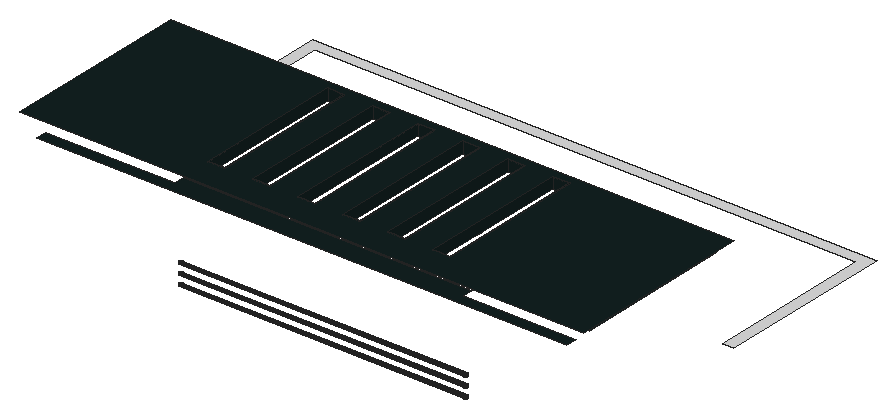
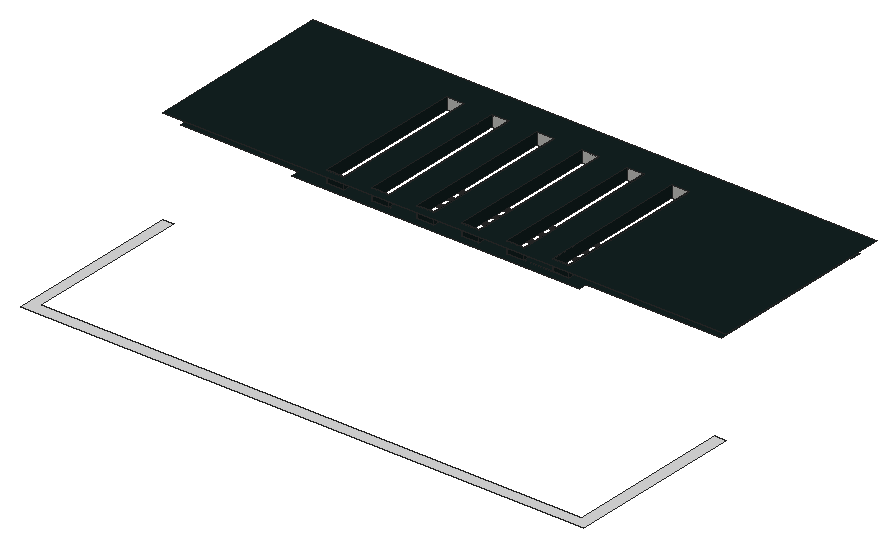
# SketchUp Ruby script. Lengths in millimetres.
U = 1.mm
M = Sketchup.active_model
def pt(a) = Geom::Point3d.new(a.map { |v| v * U })
def face(e, loops, mat)
  f = e.add_face(loops[0].map { |a| pt(a) })
  loops[1..].each { |l| e.add_face(l.map { |a| pt(a) }).erase! }
  f.material = f.back_material = mat if mat
  f
end
# faces: each face lists its corners as indices into pts; further lists are holes
def faces(e, pts, list, mat = nil) = list.each { |f| face(e, (f[0].is_a?(Array) ? f : [f]).map { |l| l.map { |i| pts[i] } }, mat) }
# xy, xz, yz: faces in a plane at the given z, y or x. An outline is a flat list of corners, or four numbers for a rectangle; further outlines are holes
def ring(l) = l.size == 4 ? [[l[0], l[1]], [l[2], l[1]], [l[2], l[3]], [l[0], l[3]]] : l.each_slice(2).to_a
def flat(e, list, mat, &to3) = list.each { |f| face(e, (f[0].is_a?(Array) ? f : [f]).map { |l| ring(l).map { |u, v| to3.(u, v) } }, mat) }
def xy(e, z, list, mat = nil) = flat(e, list, mat) { |x, y| [x, y, z] }
def xz(e, y, list, mat = nil) = flat(e, list, mat) { |x, z| [x, y, z] }
def yz(e, x, list, mat = nil) = flat(e, list, mat) { |y, z| [x, y, z] }
def lines(e, pts, list) = list.each { |a, b| e.add_line(pt(pts[a]), pt(pts[b])) }
# prism: a flat outline (further loops are holes) pulled along v
def prism(e, loops, v, mat = nil)
  f = face(e, loops, mat); d = Geom::Vector3d.new(v.map { |x| x * U })
  f.pushpull(f.normal.samedirection?(d) ? d.length : -d.length)
end
def box(e, o, s, mat = nil) = prism(e, [[o, [o[0] + s[0], o[1], o[2]], [o[0] + s[0], o[1] + s[1], o[2]], [o[0], o[1] + s[1], o[2]]]], [0, 0, s[2]], mat)
def at(x, y, z, deg = 0) = Geom::Transformation.translation(pt([x, y, z])) * Geom::Transformation.rotation(ORIGIN, Z_AXIS, deg.degrees)
def axes(o, x, y, z) = Geom::Transformation.new([*x, 0, *y, 0, *z, 0, *pt(o).to_a, 1])
def part(name) = M.definitions.add(name)
# library, detail: a bought-in or finely detailed component or shape, given as its bounding box
def library(name, o, s) = part(name).tap { |d| box(d.entities, o, s) }
def detail(e, o, s) = box(e.add_group.entities, o, s)
def put(e, d, t, mat = nil) = e.add_instance(d, t).tap { |i| i.material = mat if mat }
def group(e, t, mat = nil) = e.add_group.tap { |g| g.transformation = t; g.material = mat if mat }.entities
root = M.entities
M.materials.add("[0078_DarkSlateGray]").color = [19, 33, 33]
M.materials.add("[0128_White]").color = [252, 252, 252]
M.materials.add("[0130_Gainsboro]").color = [220, 220, 220]
xy(root,69967.5,[[7076.1,23710.9,7685.7,23710.9,7685.7,32702.5,36946.5,32702.5,36946.5,23710.9,37556.1,23710.9,37556.1,33312.1,7076.1,33312.1]],"[0130_Gainsboro]")
xy(root,74234.7,[[7990.5,13550.9,7990.5,14109.7,15000.9,14109.7,15000.9,14719.3,30545.7,14719.3,30545.7,14109.7,36641.7,14109.7,36641.7,13550.9]],"[0078_DarkSlateGray]")
xy(root,74539.5,[[[7685.7,14719.3,7685.7,23253.7,15915.3,23253.7,15915.3,15176.5,16829.7,15176.5,16829.7,23253.7,18353.7,23253.7,18353.7,15176.5,19268.1,15176.5,19268.1,23253.7,20792.1,23253.7,20792.1,15176.5,21706.5,15176.5,21706.5,23253.7,23230.5,23253.7,23230.5,15176.5,24144.9,15176.5,24144.9,23253.7,25668.9,23253.7,25668.9,15176.5,26583.3,15176.5,26583.3,23253.7,28107.3,23253.7,28107.3,15176.5,29021.7,15176.5,29021.7,23253.7,15000.9,23253.7,15000.9,23710.9,30545.7,23710.9,30545.7,23253.7,36946.5,23253.7,36946.5,14719.3],[17596.1,17794.4,17659.9,17796.3,17723.1,17804.9,17785.1,17820.1,17845.1,17841.6,17902.6,17869.3,17956.9,17902.9,18007.3,17942,18053.4,17986.1,18094.7,18034.8,18130.6,18087.5,18160.8,18143.7,18185,18202.8,18202.8,18264,18214.2,18326.8,18218.9,18390.5,18217,18454.2,18208.4,18517.5,18193.2,18579.4,18171.7,18639.5,18143.9,18697,18110.4,18751.2,18071.3,18801.7,18027.2,18847.8,17978.5,18889,17925.8,18924.9,17869.6,18955.1,17810.5,18979.3,17749.2,18997.2,17686.5,19008.5,17622.8,19013.3,17559,19011.3,17495.8,19002.7,17433.8,18987.6,17373.8,18966,17316.3,18938.3,17262,18904.7,17211.6,18865.7,17165.5,18821.6,17124.3,18772.9,17088.3,18720.1,17058.1,18663.9,17034,18604.9,17016.1,18543.6,17004.7,18480.8,17000,18417.2,17001.9,18353.4,17010.5,18290.2,17025.7,18228.2,17047.3,18168.1,17075,18110.7,17108.5,18056.4,17147.6,18006,17191.7,17959.9,17240.4,17918.6,17293.2,17882.7,17349.4,17852.5,17408.4,17828.3,17469.7,17810.5,17532.5,17799.1],[20031.3,17794.4,20095.1,17796.3,20158.3,17804.9,20220.3,17820.1,20280.4,17841.6,20337.8,17869.3,20392.1,17902.9,20442.6,17942,20488.6,17986.1,20529.9,18034.8,20565.8,18087.5,20596,18143.7,20620.2,18202.8,20638,18264,20649.4,18326.8,20654.1,18390.5,20652.2,18454.2,20643.6,18517.5,20628.4,18579.4,20606.9,18639.5,20579.2,18697,20545.6,18751.2,20506.5,18801.7,20462.4,18847.8,20413.7,18889,20361,18924.9,20304.8,18955.1,20245.7,18979.3,20184.5,18997.2,20121.7,19008.5,20058,19013.3,19994.3,19011.3,19931,19002.7,19869.1,18987.6,19809,18966,19751.5,18938.3,19697.3,18904.7,19646.8,18865.7,19600.7,18821.6,19559.5,18772.9,19523.6,18720.1,19493.4,18663.9,19469.2,18604.9,19451.3,18543.6,19440,18480.8,19435.2,18417.2,19437.2,18353.4,19445.8,18290.2,19460.9,18228.2,19482.5,18168.1,19510.2,18110.7,19543.8,18056.4,19582.8,18006,19626.9,17959.9,19675.6,17918.6,19728.4,17882.7,19784.6,17852.5,19843.6,17828.3,19904.9,17810.5,19967.7,17799.1],[24972.2,17794.4,25036,17796.3,25099.2,17804.9,25161.2,17820.1,25221.3,17841.6,25278.7,17869.3,25333,17902.9,25383.5,17942,25429.6,17986.1,25470.8,18034.8,25506.7,18087.5,25536.9,18143.7,25561.1,18202.8,25578.9,18264,25590.3,18326.8,25595,18390.5,25593.1,18454.2,25584.5,18517.5,25569.3,18579.4,25547.8,18639.5,25520.1,18697,25486.5,18751.2,25447.4,18801.7,25403.3,18847.8,25354.6,18889,25301.9,18924.9,25245.7,18955.1,25186.6,18979.3,25125.4,18997.2,25062.6,19008.5,24999,19013.3,24935.2,19011.3,24872,19002.7,24810,18987.6,24749.9,18966,24692.4,18938.3,24638.2,18904.7,24587.7,18865.7,24541.6,18821.6,24500.4,18772.9,24464.5,18720.1,24434.3,18663.9,24410.1,18604.9,24392.2,18543.6,24380.9,18480.8,24376.1,18417.2,24378.1,18353.4,24386.7,18290.2,24401.8,18228.2,24423.4,18168.1,24451.1,18110.7,24484.7,18056.4,24523.7,18006,24567.9,17959.9,24616.5,17918.6,24669.3,17882.7,24725.5,17852.5,24784.5,17828.3,24845.8,17810.5,24908.6,17799.1],[22491,17794.4,22554.7,17796.3,22618,17804.9,22679.9,17820.1,22740,17841.6,22797.5,17869.3,22851.7,17902.9,22902.2,17942,22948.3,17986.1,22989.5,18034.8,23025.4,18087.5,23055.7,18143.7,23079.8,18202.8,23097.7,18264,23109,18326.8,23113.8,18390.5,23111.8,18454.2,23103.2,18517.5,23088.1,18579.4,23066.5,18639.5,23038.8,18697,23005.2,18751.2,22966.2,18801.7,22922.1,18847.8,22873.4,18889,22820.6,18924.9,22764.4,18955.1,22705.4,18979.3,22644.1,18997.2,22581.3,19008.5,22517.7,19013.3,22453.9,19011.3,22390.7,19002.7,22328.7,18987.6,22268.7,18966,22211.2,18938.3,22156.9,18904.7,22106.5,18865.7,22060.4,18821.6,22019.1,18772.9,21983.2,18720.1,21953,18663.9,21928.8,18604.9,21911,18543.6,21899.6,18480.8,21894.9,18417.2,21896.8,18353.4,21905.4,18290.2,21920.6,18228.2,21942.1,18168.1,21969.8,18110.7,22003.4,18056.4,22042.5,18006,22086.6,17959.9,22135.3,17918.6,22188,17882.7,22244.2,17852.5,22303.3,17828.3,22364.5,17810.5,22427.3,17799.1],[27480.5,17794.4,27544.3,17796.3,27607.5,17804.9,27669.5,17820.1,27729.5,17841.6,27787,17869.3,27841.3,17902.9,27891.7,17942,27937.8,17986.1,27979,18034.8,28015,18087.5,28045.2,18143.7,28069.3,18202.8,28087.2,18264,28098.6,18326.8,28103.3,18390.5,28101.4,18454.2,28092.8,18517.5,28077.6,18579.4,28056,18639.5,28028.3,18697,27994.8,18751.2,27955.7,18801.7,27911.6,18847.8,27862.9,18889,27810.1,18924.9,27753.9,18955.1,27694.9,18979.3,27633.6,18997.2,27570.8,19008.5,27507.2,19013.3,27443.4,19011.3,27380.2,19002.7,27318.2,18987.6,27258.2,18966,27200.7,18938.3,27146.4,18904.7,27096,18865.7,27049.9,18821.6,27008.6,18772.9,26972.7,18720.1,26942.5,18663.9,26918.3,18604.9,26900.5,18543.6,26889.1,18480.8,26884.4,18417.2,26886.3,18353.4,26894.9,18290.2,26910.1,18228.2,26931.6,18168.1,26959.4,18110.7,26992.9,18056.4,27032,18006,27076.1,17959.9,27124.8,17918.6,27177.5,17882.7,27233.7,17852.5,27292.8,17828.3,27354.1,17810.5,27416.8,17799.1]]],"[0078_DarkSlateGray]")
xy(root,74539.5,[[17596.1,17794.4,17532.5,17799.1,17469.7,17810.5,17408.4,17828.3,17349.4,17852.5,17293.2,17882.7,17240.4,17918.6,17191.7,17959.9,17147.6,18006,17108.5,18056.4,17075,18110.7,17047.3,18168.1,17025.7,18228.2,17010.5,18290.2,17001.9,18353.4,17000,18417.2,17004.7,18480.8,17016.1,18543.6,17034,18604.9,17058.1,18663.9,17088.3,18720.1,17124.3,18772.9,17165.5,18821.6,17211.6,18865.7,17262,18904.7,17316.3,18938.3,17373.8,18966,17433.8,18987.6,17495.8,19002.7,17559,19011.3,17622.8,19013.3,17686.5,19008.5,17749.2,18997.2,17810.5,18979.3,17869.6,18955.1,17925.8,18924.9,17978.5,18889,18027.2,18847.8,18071.3,18801.7,18110.4,18751.2,18143.9,18697,18171.7,18639.5,18193.2,18579.4,18208.4,18517.5,18217,18454.2,18218.9,18390.5,18214.2,18326.8,18202.8,18264,18185,18202.8,18160.8,18143.7,18130.6,18087.5,18094.7,18034.8,18053.4,17986.1,18007.3,17942,17956.9,17902.9,17902.6,17869.3,17845.1,17841.6,17785.1,17820.1,17723.1,17804.9,17659.9,17796.3],[20031.3,17794.4,19967.7,17799.1,19904.9,17810.5,19843.6,17828.3,19784.6,17852.5,19728.4,17882.7,19675.6,17918.6,19626.9,17959.9,19582.8,18006,19543.8,18056.4,19510.2,18110.7,19482.5,18168.1,19460.9,18228.2,19445.8,18290.2,19437.2,18353.4,19435.2,18417.2,19440,18480.8,19451.3,18543.6,19469.2,18604.9,19493.4,18663.9,19523.6,18720.1,19559.5,18772.9,19600.7,18821.6,19646.8,18865.7,19697.3,18904.7,19751.5,18938.3,19809,18966,19869.1,18987.6,19931,19002.7,19994.3,19011.3,20058,19013.3,20121.7,19008.5,20184.5,18997.2,20245.7,18979.3,20304.8,18955.1,20361,18924.9,20413.7,18889,20462.4,18847.8,20506.5,18801.7,20545.6,18751.2,20579.2,18697,20606.9,18639.5,20628.4,18579.4,20643.6,18517.5,20652.2,18454.2,20654.1,18390.5,20649.4,18326.8,20638,18264,20620.2,18202.8,20596,18143.7,20565.8,18087.5,20529.9,18034.8,20488.6,17986.1,20442.6,17942,20392.1,17902.9,20337.8,17869.3,20280.4,17841.6,20220.3,17820.1,20158.3,17804.9,20095.1,17796.3],[22491,17794.4,22427.3,17799.1,22364.5,17810.5,22303.3,17828.3,22244.2,17852.5,22188,17882.7,22135.3,17918.6,22086.6,17959.9,22042.5,18006,22003.4,18056.4,21969.8,18110.7,21942.1,18168.1,21920.6,18228.2,21905.4,18290.2,21896.8,18353.4,21894.9,18417.2,21899.6,18480.8,21911,18543.6,21928.8,18604.9,21953,18663.9,21983.2,18720.1,22019.1,18772.9,22060.4,18821.6,22106.5,18865.7,22156.9,18904.7,22211.2,18938.3,22268.7,18966,22328.7,18987.6,22390.7,19002.7,22453.9,19011.3,22517.7,19013.3,22581.3,19008.5,22644.1,18997.2,22705.4,18979.3,22764.4,18955.1,22820.6,18924.9,22873.4,18889,22922.1,18847.8,22966.2,18801.7,23005.2,18751.2,23038.8,18697,23066.5,18639.5,23088.1,18579.4,23103.2,18517.5,23111.8,18454.2,23113.8,18390.5,23109,18326.8,23097.7,18264,23079.8,18202.8,23055.7,18143.7,23025.4,18087.5,22989.5,18034.8,22948.3,17986.1,22902.2,17942,22851.7,17902.9,22797.5,17869.3,22740,17841.6,22679.9,17820.1,22618,17804.9,22554.7,17796.3],[24972.2,17794.4,24908.6,17799.1,24845.8,17810.5,24784.5,17828.3,24725.5,17852.5,24669.3,17882.7,24616.5,17918.6,24567.9,17959.9,24523.7,18006,24484.7,18056.4,24451.1,18110.7,24423.4,18168.1,24401.8,18228.2,24386.7,18290.2,24378.1,18353.4,24376.1,18417.2,24380.9,18480.8,24392.2,18543.6,24410.1,18604.9,24434.3,18663.9,24464.5,18720.1,24500.4,18772.9,24541.6,18821.6,24587.7,18865.7,24638.2,18904.7,24692.4,18938.3,24749.9,18966,24810,18987.6,24872,19002.7,24935.2,19011.3,24999,19013.3,25062.6,19008.5,25125.4,18997.2,25186.6,18979.3,25245.7,18955.1,25301.9,18924.9,25354.6,18889,25403.3,18847.8,25447.4,18801.7,25486.5,18751.2,25520.1,18697,25547.8,18639.5,25569.3,18579.4,25584.5,18517.5,25593.1,18454.2,25595,18390.5,25590.3,18326.8,25578.9,18264,25561.1,18202.8,25536.9,18143.7,25506.7,18087.5,25470.8,18034.8,25429.6,17986.1,25383.5,17942,25333,17902.9,25278.7,17869.3,25221.3,17841.6,25161.2,17820.1,25099.2,17804.9,25036,17796.3],[27480.5,17794.4,27416.8,17799.1,27354.1,17810.5,27292.8,17828.3,27233.7,17852.5,27177.5,17882.7,27124.8,17918.6,27076.1,17959.9,27032,18006,26992.9,18056.4,26959.4,18110.7,26931.6,18168.1,26910.1,18228.2,26894.9,18290.2,26886.3,18353.4,26884.4,18417.2,26889.1,18480.8,26900.5,18543.6,26918.3,18604.9,26942.5,18663.9,26972.7,18720.1,27008.6,18772.9,27049.9,18821.6,27096,18865.7,27146.4,18904.7,27200.7,18938.3,27258.2,18966,27318.2,18987.6,27380.2,19002.7,27443.4,19011.3,27507.2,19013.3,27570.8,19008.5,27633.6,18997.2,27694.9,18979.3,27753.9,18955.1,27810.1,18924.9,27862.9,18889,27911.6,18847.8,27955.7,18801.7,27994.8,18751.2,28028.3,18697,28056,18639.5,28077.6,18579.4,28092.8,18517.5,28101.4,18454.2,28103.3,18390.5,28098.6,18326.8,28087.2,18264,28069.3,18202.8,28045.2,18143.7,28015,18087.5,27979,18034.8,27937.8,17986.1,27891.7,17942,27841.3,17902.9,27787,17869.3,27729.5,17841.6,27669.5,17820.1,27607.5,17804.9,27544.3,17796.3]],"[0128_White]")
xy(root,75149.1,[[[7076.1,13550.9,37556.1,23710.9],[28107.3,15176.5,29021.7,23253.7],[25668.9,15176.5,26583.3,23253.7],[20792.1,15176.5,21706.5,23253.7],[18353.7,15176.5,19268.1,23253.7],[23230.5,15176.5,24144.9,23253.7],[15915.3,15176.5,16829.7,23253.7]]],"[0078_DarkSlateGray]")
xz(root,14338.5,[[15000.9,69200.7,30545.7,69210.3],[15000.9,69734.1,30545.7,69743.7],[15000.9,70267.5,30545.7,70277.1]])
xz(root,14490.5,[[15000.9,69200.7,30545.7,69210.3],[15000.9,69734.1,30545.7,69743.7],[15000.9,70267.5,30545.7,70277.1]])
xz(root,15176.5,[[15915.3,74539.5,16829.7,75149.1],[18353.7,74539.5,19268.1,75149.1],[20792.1,74539.5,21706.5,75149.1],[23230.5,74539.5,24144.9,75149.1],[25668.9,74539.5,26583.3,75149.1],
  [28107.3,74539.5,29021.7,75149.1]])
xz(root,23253.7,[[15915.3,74539.5,16829.7,75149.1],[18353.7,74539.5,19268.1,75149.1],[20792.1,74539.5,21706.5,75149.1],[23230.5,74539.5,24144.9,75149.1],[25668.9,74539.5,26583.3,75149.1],
  [28107.3,74539.5,29021.7,75149.1]],"[0078_DarkSlateGray]")
yz(root,15915.3,[[15176.5,74539.5,23253.7,75149.1]],"[0078_DarkSlateGray]")
yz(root,16829.7,[[15176.5,74539.5,23253.7,75149.1]],"[0078_DarkSlateGray]")
yz(root,18353.7,[[15176.5,74539.5,23253.7,75149.1]],"[0078_DarkSlateGray]")
yz(root,19268.1,[[15176.5,74539.5,23253.7,75149.1]],"[0078_DarkSlateGray]")
yz(root,20792.1,[[15176.5,74539.5,23253.7,75149.1]],"[0078_DarkSlateGray]")
yz(root,21706.5,[[15176.5,74539.5,23253.7,75149.1]],"[0078_DarkSlateGray]")
yz(root,23230.5,[[15176.5,74539.5,23253.7,75149.1]],"[0078_DarkSlateGray]")
yz(root,24144.9,[[15176.5,74539.5,23253.7,75149.1]],"[0078_DarkSlateGray]")
yz(root,25668.9,[[15176.5,74539.5,23253.7,75149.1]],"[0078_DarkSlateGray]")
yz(root,26583.3,[[15176.5,74539.5,23253.7,75149.1]],"[0078_DarkSlateGray]")
yz(root,28107.3,[[15176.5,74539.5,23253.7,75149.1]],"[0078_DarkSlateGray]")
yz(root,29021.7,[[15176.5,74539.5,23253.7,75149.1]],"[0078_DarkSlateGray]")
p = [[15000.9,14404.9,69129.9],[15000.9,14414.5,69129.7],[30545.7,14414.5,69129.7],[30545.7,14404.9,69129.9],[15000.9,14424.1,69129.9],[30545.7,14424.1,69129.9],
  [15000.9,14395.5,69131.7],[30545.7,14395.5,69131.7],[15000.9,14433.5,69131.7],[30545.7,14433.5,69131.7],[15000.9,14386.4,69134.6],[30545.7,14386.4,69134.6],
  [15000.9,14442.6,69134.6],[30545.7,14442.6,69134.6],[15000.9,14377.8,69138.7],[30545.7,14377.8,69138.7],[15000.9,14451.2,69138.7],[30545.7,14451.2,69138.7],
  [15000.9,14369.7,69143.8],[30545.7,14369.7,69143.8],[15000.9,14459.3,69143.8],[30545.7,14459.3,69143.8],[15000.9,14362.3,69149.9],[30545.7,14362.3,69149.9],
  [15000.9,14466.7,69149.9],[30545.7,14466.7,69149.9],[15000.9,14355.8,69156.9],[30545.7,14355.8,69156.9],[15000.9,14473.2,69156.9],[30545.7,14473.2,69156.9],
  [15000.9,14350.2,69164.6],[30545.7,14350.2,69164.6],[15000.9,14478.8,69164.6],[30545.7,14478.8,69164.6],[15000.9,14345.6,69173],[30545.7,14345.6,69173],
  [15000.9,14483.4,69173],[30545.7,14483.4,69173],[15000.9,14342,69181.9],[30545.7,14342,69181.9],[15000.9,14487,69181.9],[30545.7,14487,69181.9],
  [15000.9,14339.6,69191.2],[30545.7,14339.6,69191.2],[15000.9,14489.4,69191.2],[30545.7,14489.4,69191.2],[15000.9,14338.5,69200.7],[30545.7,14338.5,69200.7],
  [15000.9,14490.5,69200.7],[30545.7,14490.5,69200.7],[15000.9,14339.6,69219.8],[15000.9,14338.5,69210.3],[30545.7,14338.5,69210.3],[30545.7,14339.6,69219.8],
  [15000.9,14490.5,69210.3],[15000.9,14489.4,69219.8],[30545.7,14489.4,69219.8],[30545.7,14490.5,69210.3],[15000.9,14342,69229],[30545.7,14342,69229],
  [15000.9,14487,69229],[30545.7,14487,69229],[15000.9,14345.6,69237.9],[30545.7,14345.6,69237.9],[15000.9,14483.4,69237.9],[30545.7,14483.4,69237.9],
  [15000.9,14350.2,69246.3],[30545.7,14350.2,69246.3],[15000.9,14478.8,69246.3],[30545.7,14478.8,69246.3],[15000.9,14355.8,69254],[30545.7,14355.8,69254],
  [15000.9,14473.2,69254],[30545.7,14473.2,69254],[15000.9,14362.3,69261],[30545.7,14362.3,69261],[15000.9,14466.7,69261],[30545.7,14466.7,69261],
  [15000.9,14369.7,69267.1],[30545.7,14369.7,69267.1],[15000.9,14459.3,69267.1],[30545.7,14459.3,69267.1],[15000.9,14377.8,69272.2],[30545.7,14377.8,69272.2],
  [15000.9,14451.2,69272.2],[30545.7,14451.2,69272.2],[15000.9,14386.4,69276.3],[30545.7,14386.4,69276.3],[15000.9,14442.6,69276.3],[30545.7,14442.6,69276.3],
  [15000.9,14395.5,69279.3],[30545.7,14395.5,69279.3],[15000.9,14433.5,69279.3],[30545.7,14433.5,69279.3],[15000.9,14404.9,69281.1],[30545.7,14404.9,69281.1],
  [15000.9,14424.1,69281.1],[30545.7,14424.1,69281.1],[15000.9,14414.5,69281.7],[30545.7,14414.5,69281.7],[15000.9,14404.9,69663.3],[15000.9,14414.5,69663.1],
  [30545.7,14414.5,69663.1],[30545.7,14404.9,69663.3],[15000.9,14424.1,69663.3],[30545.7,14424.1,69663.3],[15000.9,14395.5,69665.1],[30545.7,14395.5,69665.1],
  [15000.9,14433.5,69665.1],[30545.7,14433.5,69665.1],[15000.9,14386.4,69668],[30545.7,14386.4,69668],[15000.9,14442.6,69668],[30545.7,14442.6,69668],
  [15000.9,14377.8,69672.1],[30545.7,14377.8,69672.1],[15000.9,14451.2,69672.1],[30545.7,14451.2,69672.1],[15000.9,14369.7,69677.2],[30545.7,14369.7,69677.2],
  [15000.9,14459.3,69677.2],[30545.7,14459.3,69677.2],[15000.9,14362.3,69683.3],[30545.7,14362.3,69683.3],[15000.9,14466.7,69683.3],[30545.7,14466.7,69683.3],
  [15000.9,14355.8,69690.3],[30545.7,14355.8,69690.3],[15000.9,14473.2,69690.3],[30545.7,14473.2,69690.3],[15000.9,14350.2,69698],[30545.7,14350.2,69698],
  [15000.9,14478.8,69698],[30545.7,14478.8,69698],[15000.9,14345.6,69706.4],[30545.7,14345.6,69706.4],[15000.9,14483.4,69706.4],[30545.7,14483.4,69706.4],
  [15000.9,14342,69715.3],[30545.7,14342,69715.3],[15000.9,14487,69715.3],[30545.7,14487,69715.3],[15000.9,14339.6,69724.6],[30545.7,14339.6,69724.6],
  [15000.9,14489.4,69724.6],[30545.7,14489.4,69724.6],[15000.9,14338.5,69734.1],[30545.7,14338.5,69734.1],[15000.9,14490.5,69734.1],[30545.7,14490.5,69734.1],
  [15000.9,14339.6,69753.2],[15000.9,14338.5,69743.7],[30545.7,14338.5,69743.7],[30545.7,14339.6,69753.2],[15000.9,14490.5,69743.7],[15000.9,14489.4,69753.2],
  [30545.7,14489.4,69753.2],[30545.7,14490.5,69743.7],[15000.9,14342,69762.4],[30545.7,14342,69762.4],[15000.9,14487,69762.4],[30545.7,14487,69762.4],
  [15000.9,14345.6,69771.3],[30545.7,14345.6,69771.3],[15000.9,14483.4,69771.3],[30545.7,14483.4,69771.3],[15000.9,14350.2,69779.7],[30545.7,14350.2,69779.7],
  [15000.9,14478.8,69779.7],[30545.7,14478.8,69779.7],[15000.9,14355.8,69787.4],[30545.7,14355.8,69787.4],[15000.9,14473.2,69787.4],[30545.7,14473.2,69787.4],
  [15000.9,14362.3,69794.4],[30545.7,14362.3,69794.4],[15000.9,14466.7,69794.4],[30545.7,14466.7,69794.4],[15000.9,14369.7,69800.5],[30545.7,14369.7,69800.5],
  [15000.9,14459.3,69800.5],[30545.7,14459.3,69800.5],[15000.9,14377.8,69805.6],[30545.7,14377.8,69805.6],[15000.9,14451.2,69805.6],[30545.7,14451.2,69805.6],
  [15000.9,14386.4,69809.7],[30545.7,14386.4,69809.7],[15000.9,14442.6,69809.7],[30545.7,14442.6,69809.7],[15000.9,14395.5,69812.7],[30545.7,14395.5,69812.7],
  [15000.9,14433.5,69812.7],[30545.7,14433.5,69812.7],[15000.9,14404.9,69814.5],[30545.7,14404.9,69814.5],[15000.9,14424.1,69814.5],[30545.7,14424.1,69814.5],
  [15000.9,14414.5,69815.1],[30545.7,14414.5,69815.1],[15000.9,14404.9,70196.7],[15000.9,14414.5,70196.5],[30545.7,14414.5,70196.5],[30545.7,14404.9,70196.7],
  [15000.9,14424.1,70196.7],[30545.7,14424.1,70196.7],[15000.9,14395.5,70198.5],[30545.7,14395.5,70198.5],[15000.9,14433.5,70198.5],[30545.7,14433.5,70198.5],
  [15000.9,14386.4,70201.4],[30545.7,14386.4,70201.4],[15000.9,14442.6,70201.4],[30545.7,14442.6,70201.4],[15000.9,14377.8,70205.5],[30545.7,14377.8,70205.5],
  [15000.9,14451.2,70205.5],[30545.7,14451.2,70205.5],[15000.9,14369.7,70210.6],[30545.7,14369.7,70210.6],[15000.9,14459.3,70210.6],[30545.7,14459.3,70210.6],
  [15000.9,14362.3,70216.7],[30545.7,14362.3,70216.7],[15000.9,14466.7,70216.7],[30545.7,14466.7,70216.7],[15000.9,14355.8,70223.7],[30545.7,14355.8,70223.7],
  [15000.9,14473.2,70223.7],[30545.7,14473.2,70223.7],[15000.9,14350.2,70231.4],[30545.7,14350.2,70231.4],[15000.9,14478.8,70231.4],[30545.7,14478.8,70231.4],
  [15000.9,14345.6,70239.8],[30545.7,14345.6,70239.8],[15000.9,14483.4,70239.8],[30545.7,14483.4,70239.8],[15000.9,14342,70248.7],[30545.7,14342,70248.7],
  [15000.9,14487,70248.7],[30545.7,14487,70248.7],[15000.9,14339.6,70258],[30545.7,14339.6,70258],[15000.9,14489.4,70258],[30545.7,14489.4,70258],
  [15000.9,14338.5,70267.5],[30545.7,14338.5,70267.5],[15000.9,14490.5,70267.5],[30545.7,14490.5,70267.5],[15000.9,14339.6,70286.6],[15000.9,14338.5,70277.1],
  [30545.7,14338.5,70277.1],[30545.7,14339.6,70286.6],[15000.9,14490.5,70277.1],[15000.9,14489.4,70286.6],[30545.7,14489.4,70286.6],[30545.7,14490.5,70277.1],
  [15000.9,14342,70295.8],[30545.7,14342,70295.8],[15000.9,14487,70295.8],[30545.7,14487,70295.8],[15000.9,14345.6,70304.7],[30545.7,14345.6,70304.7],
  [15000.9,14483.4,70304.7],[30545.7,14483.4,70304.7],[15000.9,14350.2,70313.1],[30545.7,14350.2,70313.1],[15000.9,14478.8,70313.1],[30545.7,14478.8,70313.1],
  [15000.9,14355.8,70320.8],[30545.7,14355.8,70320.8],[15000.9,14473.2,70320.8],[30545.7,14473.2,70320.8],[15000.9,14362.3,70327.8],[30545.7,14362.3,70327.8],
  [15000.9,14466.7,70327.8],[30545.7,14466.7,70327.8],[15000.9,14369.7,70333.9],[30545.7,14369.7,70333.9],[15000.9,14459.3,70333.9],[30545.7,14459.3,70333.9],
  [15000.9,14377.8,70339],[30545.7,14377.8,70339],[15000.9,14451.2,70339],[30545.7,14451.2,70339],[15000.9,14386.4,70343.1],[30545.7,14386.4,70343.1],
  [15000.9,14442.6,70343.1],[30545.7,14442.6,70343.1],[15000.9,14395.5,70346.1],[30545.7,14395.5,70346.1],[15000.9,14433.5,70346.1],[30545.7,14433.5,70346.1],
  [15000.9,14404.9,70347.9],[30545.7,14404.9,70347.9],[15000.9,14424.1,70347.9],[30545.7,14424.1,70347.9],[15000.9,14414.5,70348.5],[30545.7,14414.5,70348.5]]
faces(root,p,[[0,1,2,3],[1,4,5,2],[6,0,3,7],[4,8,9,5],[10,6,7,11],[8,12,13,9],[14,10,11,15],[12,16,17,13],
  [18,14,15,19],[16,20,21,17],[22,18,19,23],[20,24,25,21],[26,22,23,27],[24,28,29,25],[30,26,27,31],[28,32,33,29],
  [34,30,31,35],[32,36,37,33],[38,34,35,39],[36,40,41,37],[42,38,39,43],[40,44,45,41],[46,42,43,47],[44,48,49,45],
  [50,51,52,53],[54,55,56,57],[58,50,53,59],[55,60,61,56],[62,58,59,63],[60,64,65,61],[66,62,63,67],[64,68,69,65],
  [70,66,67,71],[68,72,73,69],[74,70,71,75],[72,76,77,73],[78,74,75,79],[76,80,81,77],[82,78,79,83],[80,84,85,81],
  [86,82,83,87],[84,88,89,85],[90,86,87,91],[88,92,93,89],[94,90,91,95],[92,96,97,93],[98,94,95,99],[96,98,99,97],
  [100,101,102,103],[101,104,105,102],[106,100,103,107],[104,108,109,105],[110,106,107,111],[108,112,113,109],[114,110,111,115],[112,116,117,113],
  [118,114,115,119],[116,120,121,117],[122,118,119,123],[120,124,125,121],[126,122,123,127],[124,128,129,125],[130,126,127,131],[128,132,133,129],
  [134,130,131,135],[132,136,137,133],[138,134,135,139],[136,140,141,137],[142,138,139,143],[140,144,145,141],[146,142,143,147],[144,148,149,145],
  [150,151,152,153],[154,155,156,157],[158,150,153,159],[155,160,161,156],[162,158,159,163],[160,164,165,161],[166,162,163,167],[164,168,169,165],
  [170,166,167,171],[168,172,173,169],[174,170,171,175],[172,176,177,173],[178,174,175,179],[176,180,181,177],[182,178,179,183],[180,184,185,181],
  [186,182,183,187],[184,188,189,185],[190,186,187,191],[188,192,193,189],[194,190,191,195],[192,196,197,193],[198,194,195,199],[196,198,199,197],
  [200,201,202,203],[201,204,205,202],[206,200,203,207],[204,208,209,205],[210,206,207,211],[208,212,213,209],[214,210,211,215],[212,216,217,213],
  [218,214,215,219],[216,220,221,217],[222,218,219,223],[220,224,225,221],[226,222,223,227],[224,228,229,225],[230,226,227,231],[228,232,233,229],
  [234,230,231,235],[232,236,237,233],[238,234,235,239],[236,240,241,237],[242,238,239,243],[240,244,245,241],[246,242,243,247],[244,248,249,245],
  [250,251,252,253],[254,255,256,257],[258,250,253,259],[255,260,261,256],[262,258,259,263],[260,264,265,261],[266,262,263,267],[264,268,269,265],
  [270,266,267,271],[268,272,273,269],[274,270,271,275],[272,276,277,273],[278,274,275,279],[276,280,281,277],[282,278,279,283],[280,284,285,281],
  [286,282,283,287],[284,288,289,285],[290,286,287,291],[288,292,293,289],[294,290,291,295],[292,296,297,293],[298,294,295,299],[296,298,299,297]])
